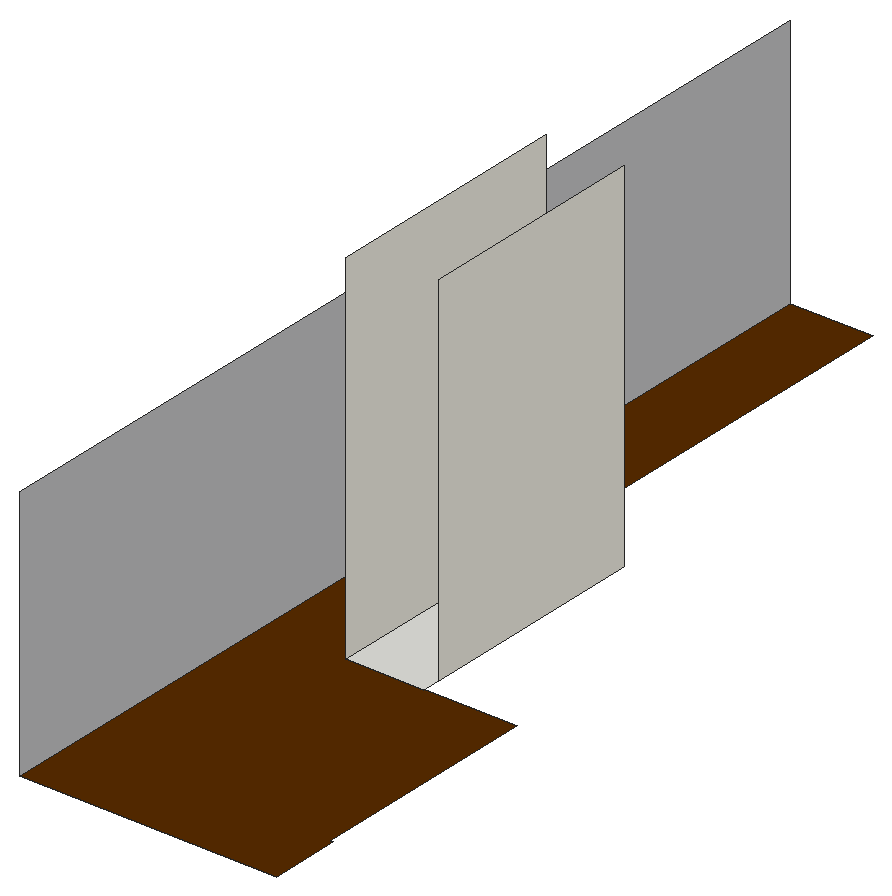
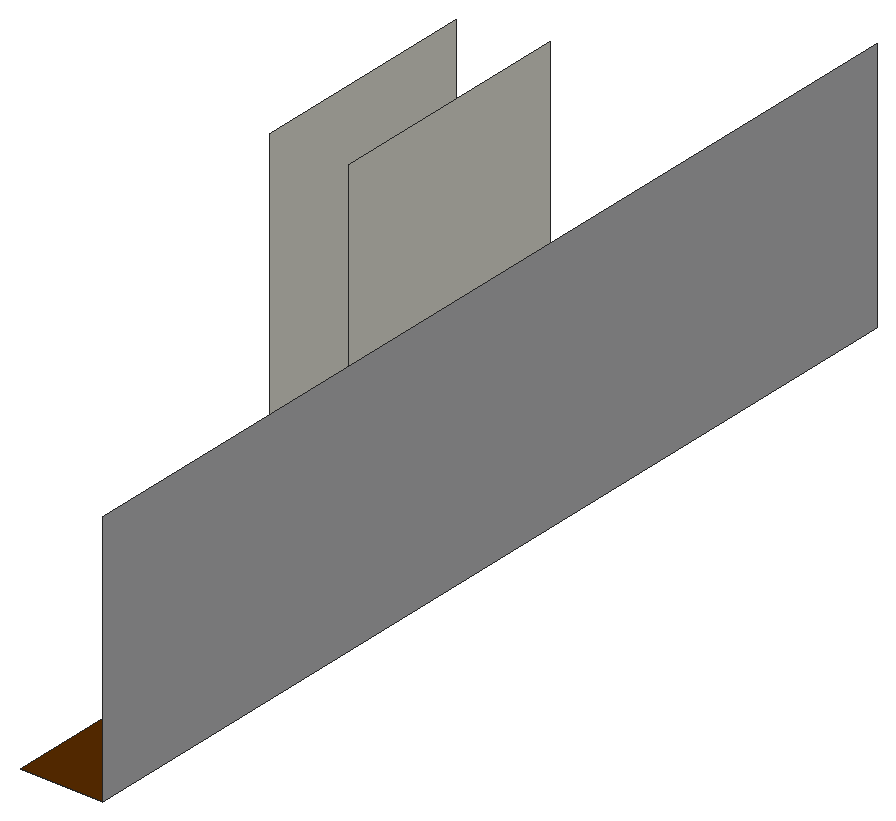
# SketchUp Ruby script. Lengths in inches.
U = 1.inch
M = Sketchup.active_model
def pt(a) = Geom::Point3d.new(a.map { |v| v * U })
def face(e, loops, mat)
  f = e.add_face(loops[0].map { |a| pt(a) })
  loops[1..].each { |l| e.add_face(l.map { |a| pt(a) }).erase! }
  f.material = f.back_material = mat if mat
  f
end
# faces: each face lists its corners as indices into pts; further lists are holes
def faces(e, pts, list, mat = nil) = list.each { |f| face(e, (f[0].is_a?(Array) ? f : [f]).map { |l| l.map { |i| pts[i] } }, mat) }
# xy, xz, yz: faces in a plane at the given z, y or x. An outline is a flat list of corners, or four numbers for a rectangle; further outlines are holes
def ring(l) = l.size == 4 ? [[l[0], l[1]], [l[2], l[1]], [l[2], l[3]], [l[0], l[3]]] : l.each_slice(2).to_a
def flat(e, list, mat, &to3) = list.each { |f| face(e, (f[0].is_a?(Array) ? f : [f]).map { |l| ring(l).map { |u, v| to3.(u, v) } }, mat) }
def xy(e, z, list, mat = nil) = flat(e, list, mat) { |x, y| [x, y, z] }
def xz(e, y, list, mat = nil) = flat(e, list, mat) { |x, z| [x, y, z] }
def yz(e, x, list, mat = nil) = flat(e, list, mat) { |y, z| [x, y, z] }
def lines(e, pts, list) = list.each { |a, b| e.add_line(pt(pts[a]), pt(pts[b])) }
# prism: a flat outline (further loops are holes) pulled along v
def prism(e, loops, v, mat = nil)
  f = face(e, loops, mat); d = Geom::Vector3d.new(v.map { |x| x * U })
  f.pushpull(f.normal.samedirection?(d) ? d.length : -d.length)
end
def box(e, o, s, mat = nil) = prism(e, [[o, [o[0] + s[0], o[1], o[2]], [o[0] + s[0], o[1] + s[1], o[2]], [o[0], o[1] + s[1], o[2]]]], [0, 0, s[2]], mat)
def at(x, y, z, deg = 0) = Geom::Transformation.translation(pt([x, y, z])) * Geom::Transformation.rotation(ORIGIN, Z_AXIS, deg.degrees)
def axes(o, x, y, z) = Geom::Transformation.new([*x, 0, *y, 0, *z, 0, *pt(o).to_a, 1])
def part(name) = M.definitions.add(name)
# library, detail: a bought-in or finely detailed component or shape, given as its bounding box
def library(name, o, s) = part(name).tap { |d| box(d.entities, o, s) }
def detail(e, o, s) = box(e.add_group.entities, o, s)
def put(e, d, t, mat = nil) = e.add_instance(d, t).tap { |i| i.material = mat if mat }
def group(e, t, mat = nil) = e.add_group.tap { |g| g.transformation = t; g.material = mat if mat }.entities
root = M.entities
M.materials.add("[Color C07]").color = [89, 44, 0]
M.materials.add("[Fencing Metal Straight]").color = [194, 195, 196]
M.materials.add("[Tile Limestone Large]").color = [237, 234, 224]
xy(root,17.625,[[46.1875,137.79,76.4,233.86]])
xy(root,17.625,[[14.48,21.02,113.3,21.02,113.3,47.98,111.93,47.98,111.93,137.79,46.1875,137.79,46.1875,390.99,14.48,390.99]],"[Color C07]")
yz(root,14.48,[[21.02,17.625,390.99,115.1875]],"[Fencing Metal Straight]")
yz(root,46.1875,[[137.79,17.625,233.86,155.84]],"[Tile Limestone Large]")
yz(root,76.4,[[144.7,17.625,233.86,155.84]],"[Tile Limestone Large]")
